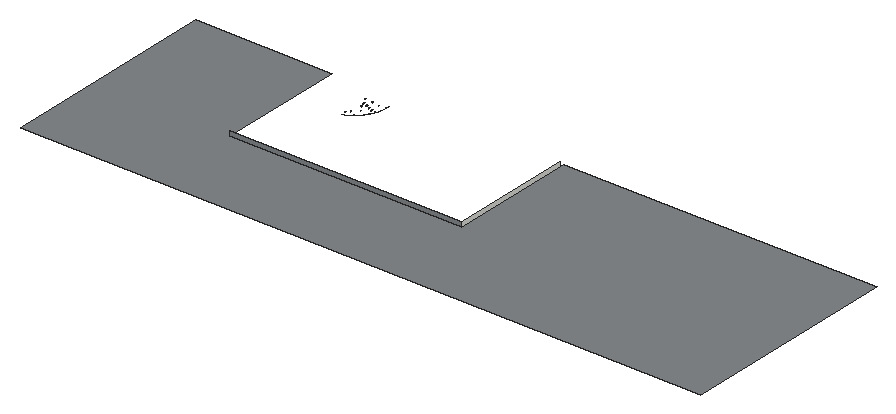
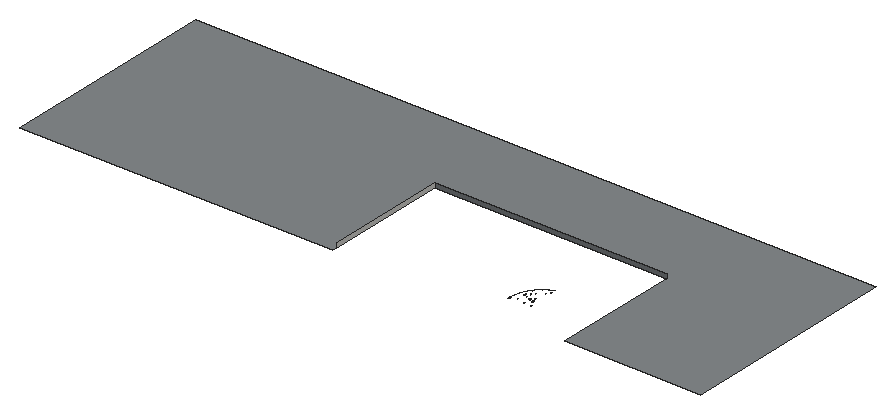
# SketchUp Ruby script. Lengths in inches.
U = 1.inch
M = Sketchup.active_model
def pt(a) = Geom::Point3d.new(a.map { |v| v * U })
def face(e, loops, mat)
  f = e.add_face(loops[0].map { |a| pt(a) })
  loops[1..].each { |l| e.add_face(l.map { |a| pt(a) }).erase! }
  f.material = f.back_material = mat if mat
  f
end
# faces: each face lists its corners as indices into pts; further lists are holes
def faces(e, pts, list, mat = nil) = list.each { |f| face(e, (f[0].is_a?(Array) ? f : [f]).map { |l| l.map { |i| pts[i] } }, mat) }
# xy, xz, yz: faces in a plane at the given z, y or x. An outline is a flat list of corners, or four numbers for a rectangle; further outlines are holes
def ring(l) = l.size == 4 ? [[l[0], l[1]], [l[2], l[1]], [l[2], l[3]], [l[0], l[3]]] : l.each_slice(2).to_a
def flat(e, list, mat, &to3) = list.each { |f| face(e, (f[0].is_a?(Array) ? f : [f]).map { |l| ring(l).map { |u, v| to3.(u, v) } }, mat) }
def xy(e, z, list, mat = nil) = flat(e, list, mat) { |x, y| [x, y, z] }
def xz(e, y, list, mat = nil) = flat(e, list, mat) { |x, z| [x, y, z] }
def yz(e, x, list, mat = nil) = flat(e, list, mat) { |y, z| [x, y, z] }
def lines(e, pts, list) = list.each { |a, b| e.add_line(pt(pts[a]), pt(pts[b])) }
# prism: a flat outline (further loops are holes) pulled along v
def prism(e, loops, v, mat = nil)
  f = face(e, loops, mat); d = Geom::Vector3d.new(v.map { |x| x * U })
  f.pushpull(f.normal.samedirection?(d) ? d.length : -d.length)
end
def box(e, o, s, mat = nil) = prism(e, [[o, [o[0] + s[0], o[1], o[2]], [o[0] + s[0], o[1] + s[1], o[2]], [o[0], o[1] + s[1], o[2]]]], [0, 0, s[2]], mat)
def at(x, y, z, deg = 0) = Geom::Transformation.translation(pt([x, y, z])) * Geom::Transformation.rotation(ORIGIN, Z_AXIS, deg.degrees)
def axes(o, x, y, z) = Geom::Transformation.new([*x, 0, *y, 0, *z, 0, *pt(o).to_a, 1])
def part(name) = M.definitions.add(name)
# library, detail: a bought-in or finely detailed component or shape, given as its bounding box
def library(name, o, s) = part(name).tap { |d| box(d.entities, o, s) }
def detail(e, o, s) = box(e.add_group.entities, o, s)
def put(e, d, t, mat = nil) = e.add_instance(d, t).tap { |i| i.material = mat if mat }
def group(e, t, mat = nil) = e.add_group.tap { |g| g.transformation = t; g.material = mat if mat }.entities
root = M.entities
M.materials.add("[Asphalt_Stamped_Brick]").color = [149, 133, 134]
M.materials.add("[Blacktop Old 01]").color = [132, 136, 139]
M.materials.add("[Metal_Steel_Textured_White]").color = [191, 191, 191]
xy(root,0,[[4.25,0,4.25,181.5,116.615,181.5,116.615,76.29,308.325,76.29,308.325,181.5,566.5625,181.5,566.5625,0]],"[Blacktop Old 01]")
xy(root,3.625,[[165.877,142.641,165.872,142.643,165.868,142.647,165.865,142.651,165.863,142.656,165.862,142.661,165.863,142.666,165.865,142.671,165.868,142.675,165.872,142.678,165.877,142.68,165.882,142.681,165.887,142.68,165.892,142.678,165.896,142.675,165.899,142.671,165.901,142.666,165.902,142.661,165.901,142.656,165.899,142.651,165.896,142.647,165.892,142.643,165.887,142.641],[170.535,147.293,170.529,147.294,170.525,147.296,170.521,147.299,170.517,147.303,170.515,147.308,170.515,147.318,170.517,147.323,170.521,147.327,170.525,147.33,170.529,147.332,170.535,147.333,170.54,147.332,170.545,147.33,170.549,147.327,170.552,147.323,170.554,147.318,170.555,147.313,170.554,147.308,170.552,147.303,170.549,147.299,170.545,147.296,170.54,147.294],[162.784,154.587,162.779,154.588,162.774,154.59,162.77,154.593,162.767,154.597,162.765,154.602,162.764,154.607,162.765,154.613,162.767,154.617,162.77,154.621,162.774,154.625,162.779,154.627,162.789,154.627,162.794,154.625,162.798,154.621,162.801,154.617,162.803,154.613,162.804,154.607,162.803,154.602,162.801,154.597,162.798,154.593,162.794,154.59,162.789,154.588],[162.103,155.035,162.097,155.036,162.093,155.038,162.089,155.041,162.085,155.045,162.083,155.05,162.083,155.06,162.085,155.065,162.089,155.069,162.093,155.072,162.097,155.074,162.103,155.075,162.108,155.074,162.113,155.072,162.117,155.069,162.12,155.065,162.122,155.06,162.123,155.055,162.122,155.05,162.12,155.045,162.117,155.041,162.113,155.038,162.108,155.036],[168.183,156.181,168.178,156.183,168.174,156.186,168.17,156.191,168.168,156.195,168.168,156.206,168.17,156.21,168.174,156.215,168.178,156.218,168.183,156.22,168.193,156.22,168.198,156.218,168.202,156.215,168.205,156.21,168.207,156.206,168.208,156.2,168.207,156.195,168.205,156.191,168.202,156.186,168.198,156.183,168.193,156.181],
  [165.188,157.423,165.183,157.424,165.178,157.426,165.174,157.429,165.171,157.433,165.169,157.438,165.168,157.443,165.169,157.448,165.171,157.453,165.174,157.457,165.178,157.46,165.183,157.462,165.188,157.463,165.193,157.462,165.198,157.46,165.202,157.457,165.205,157.453,165.207,157.448,165.208,157.443,165.207,157.438,165.205,157.433,165.202,157.429,165.198,157.426,165.193,157.424],[161.18,158.219,161.175,158.22,161.17,158.222,161.166,158.225,161.163,158.229,161.161,158.234,161.16,158.239,161.161,158.244,161.163,158.249,161.166,158.253,161.17,158.256,161.175,158.258,161.18,158.259,161.185,158.258,161.19,158.256,161.194,158.253,161.197,158.249,161.199,158.244,161.2,158.239,161.199,158.234,161.197,158.229,161.194,158.225,161.19,158.222,161.185,158.22],[161.48,158.957,161.476,158.959,161.471,158.963,161.468,158.967,161.466,158.971,161.466,158.982,161.468,158.987,161.471,158.991,161.476,158.994,161.48,158.996,161.486,158.997,161.491,158.996,161.496,158.994,161.5,158.991,161.503,158.987,161.505,158.982,161.506,158.977,161.505,158.971,161.503,158.967,161.5,158.963,161.496,158.959,161.491,158.957]],"[Asphalt_Stamped_Brick]")
xy(root,3.625,[[[159.48,138.919,159.457,138.922,159.436,138.931,159.417,138.945,159.403,138.963,159.394,138.985,159.391,139.008,159.394,139.031,159.403,139.052,159.417,139.071,159.436,139.085,159.457,139.094,159.48,139.097,159.503,139.094,159.525,139.085,159.543,139.071,159.557,139.052,159.566,139.031,159.569,139.008,159.566,138.985,159.557,138.963,159.543,138.945,159.525,138.931,159.503,138.922],[159.48,138.92,159.503,138.923,159.524,138.932,159.542,138.945,159.556,138.964,159.565,138.985,159.568,139.008,159.565,139.03,159.556,139.052,159.542,139.07,159.524,139.084,159.503,139.093,159.48,139.096,159.457,139.093,159.436,139.084,159.418,139.07,159.404,139.052,159.395,139.03,159.392,139.008,159.395,138.985,159.404,138.964,159.418,138.945,159.436,138.932,159.457,138.923]],[[160.218,139.224,160.195,139.227,160.173,139.236,160.155,139.25,160.141,139.269,160.132,139.29,160.129,139.313,160.132,139.336,160.141,139.358,160.155,139.376,160.173,139.39,160.195,139.399,160.218,139.402,160.241,139.399,160.262,139.39,160.281,139.376,160.295,139.358,160.304,139.336,160.307,139.313,160.304,139.29,160.295,139.269,160.281,139.25,160.262,139.236,160.241,139.227],[160.218,139.225,160.24,139.228,160.262,139.237,160.28,139.251,160.294,139.269,160.303,139.29,160.306,139.313,160.303,139.336,160.294,139.357,160.28,139.375,160.262,139.389,160.24,139.398,160.218,139.401,160.195,139.398,160.174,139.389,160.156,139.375,160.142,139.357,160.133,139.336,160.13,139.313,160.133,139.29,160.142,139.269,160.156,139.251,160.174,139.237,160.195,139.228]],[[163.155,140.772,163.146,140.773,163.137,140.777,163.13,140.783,163.124,140.79,163.12,140.799,163.119,140.809,163.12,140.818,163.124,140.827,163.13,140.834,163.137,140.84,163.146,140.844,163.155,140.845,163.165,140.844,163.174,140.84,163.181,140.834,163.187,140.827,163.191,140.818,163.192,140.809,163.191,140.799,163.187,140.79,163.181,140.783,163.174,140.777,163.165,140.773],[163.15,140.789,163.161,140.789,163.165,140.791,163.169,140.794,163.173,140.799,163.175,140.803,163.175,140.814,163.173,140.819,163.169,140.823,163.165,140.826,163.161,140.828,163.15,140.828,163.145,140.826,163.141,140.823,163.138,140.819,163.136,140.814,163.135,140.809,163.136,140.803,163.138,140.799,163.141,140.794,163.145,140.791]],[[158.975,142.224,158.952,142.227,158.931,142.236,158.912,142.25,158.898,142.269,158.889,142.29,158.886,142.313,158.889,142.336,158.898,142.358,158.912,142.376,158.931,142.39,158.952,142.399,158.975,142.402,158.998,142.399,159.02,142.39,159.038,142.376,159.052,142.358,159.061,142.336,159.064,142.313,159.061,142.29,159.052,142.269,159.038,142.25,159.02,142.236,158.998,142.227],[158.975,142.225,158.998,142.228,159.019,142.237,159.037,142.251,159.051,142.269,159.06,142.29,159.063,142.313,159.06,142.336,159.051,142.357,159.037,142.375,159.019,142.389,158.998,142.398,158.975,142.401,158.952,142.398,158.931,142.389,158.913,142.375,158.899,142.357,158.89,142.336,158.887,142.313,158.89,142.29,158.899,142.269,158.913,142.251,158.931,142.237,158.952,142.228]],[[165.882,142.624,165.873,142.625,165.864,142.629,165.856,142.635,165.85,142.642,165.847,142.651,165.846,142.661,165.847,142.67,165.85,142.679,165.856,142.687,165.864,142.692,165.873,142.696,165.882,142.697,165.892,142.696,165.9,142.692,165.908,142.687,165.914,142.679,165.917,142.67,165.919,142.661,165.917,142.651,165.914,142.642,165.908,142.635,165.9,142.629,165.892,142.625],[165.877,142.641,165.887,142.641,165.892,142.643,165.896,142.647,165.899,142.651,165.901,142.656,165.902,142.661,165.901,142.666,165.899,142.671,165.896,142.675,165.892,142.678,165.887,142.68,165.882,142.681,165.877,142.68,165.872,142.678,165.868,142.675,165.865,142.671,165.863,142.666,165.862,142.661,165.863,142.656,165.865,142.651,165.868,142.647,165.872,142.643]],
  [[168.355,144.751,168.332,144.755,168.31,144.763,168.292,144.778,168.278,144.796,168.269,144.817,168.266,144.84,168.269,144.863,168.278,144.885,168.292,144.903,168.31,144.917,168.332,144.926,168.355,144.929,168.378,144.926,168.399,144.917,168.418,144.903,168.432,144.885,168.441,144.863,168.444,144.84,168.441,144.817,168.432,144.796,168.418,144.778,168.399,144.763,168.378,144.755],[168.355,144.752,168.378,144.755,168.399,144.764,168.417,144.778,168.431,144.796,168.44,144.818,168.443,144.84,168.44,144.863,168.431,144.884,168.417,144.903,168.399,144.917,168.378,144.925,168.355,144.928,168.332,144.925,168.311,144.917,168.293,144.903,168.279,144.884,168.27,144.863,168.267,144.84,168.27,144.818,168.279,144.796,168.293,144.778,168.311,144.764,168.332,144.755]],[[161.174,144.911,161.151,144.914,161.13,144.922,161.111,144.936,161.097,144.955,161.089,144.976,161.086,144.999,161.089,145.021,161.097,145.043,161.111,145.061,161.13,145.075,161.151,145.083,161.174,145.086,161.196,145.083,161.218,145.075,161.236,145.061,161.25,145.043,161.258,145.021,161.261,144.999,161.258,144.976,161.25,144.955,161.236,144.936,161.218,144.922,161.196,144.914],[161.174,144.962,161.183,144.963,161.192,144.967,161.199,144.973,161.205,144.98,161.209,144.989,161.21,144.999,161.209,145.008,161.205,145.017,161.199,145.024,161.192,145.03,161.183,145.034,161.174,145.035,161.164,145.034,161.155,145.03,161.148,145.024,161.142,145.017,161.138,145.008,161.137,144.999,161.138,144.989,161.142,144.98,161.148,144.973,161.155,144.967,161.164,144.963]],[[161.174,144.962,161.164,144.963,161.155,144.967,161.148,144.973,161.142,144.98,161.138,144.989,161.137,144.999,161.138,145.008,161.142,145.017,161.148,145.024,161.155,145.03,161.164,145.034,161.174,145.035,161.183,145.034,161.192,145.03,161.199,145.024,161.205,145.017,161.209,145.008,161.21,144.999,161.209,144.989,161.205,144.98,161.199,144.973,161.192,144.967,161.183,144.963],[161.168,144.979,161.179,144.979,161.184,144.981,161.1875,144.984,161.191,144.989,161.193,144.993,161.194,144.999,161.193,145.004,161.191,145.009,161.1875,145.013,161.184,145.016,161.179,145.018,161.174,145.019,161.168,145.018,161.164,145.016,161.159,145.013,161.156,145.009,161.154,145.004,161.154,144.993,161.156,144.989,161.159,144.984,161.164,144.981]],[161.168,144.979,161.164,144.981,161.159,144.984,161.156,144.989,161.154,144.993,161.154,145.004,161.156,145.009,161.159,145.013,161.164,145.016,161.168,145.018,161.174,145.019,161.179,145.018,161.184,145.016,161.1875,145.013,161.191,145.009,161.193,145.004,161.194,144.999,161.193,144.993,161.191,144.989,161.1875,144.984,161.184,144.981,161.179,144.979],[[170.535,147.225,170.512,147.228,170.491,147.237,170.472,147.251,170.458,147.269,170.45,147.29,170.447,147.313,170.45,147.336,170.458,147.357,170.472,147.375,170.491,147.389,170.512,147.398,170.535,147.401,170.557,147.398,170.579,147.389,170.597,147.375,170.611,147.357,170.62,147.336,170.623,147.313,170.62,147.29,170.611,147.269,170.597,147.251,170.579,147.237,170.557,147.228],[170.535,147.277,170.544,147.278,170.553,147.281,170.561,147.287,170.566,147.295,170.57,147.304,170.571,147.313,170.57,147.323,170.566,147.331,170.561,147.339,170.553,147.345,170.544,147.349,170.535,147.35,170.525,147.349,170.516,147.345,170.509,147.339,170.503,147.331,170.499,147.323,170.498,147.313,170.499,147.304,170.503,147.295,170.509,147.287,170.516,147.281,170.525,147.278]],
  [[170.535,147.277,170.525,147.278,170.516,147.281,170.509,147.287,170.503,147.295,170.499,147.304,170.498,147.313,170.499,147.323,170.503,147.331,170.509,147.339,170.516,147.345,170.525,147.349,170.535,147.35,170.544,147.349,170.553,147.345,170.561,147.339,170.566,147.331,170.57,147.323,170.571,147.313,170.57,147.304,170.566,147.295,170.561,147.287,170.553,147.281,170.544,147.278],[170.535,147.293,170.54,147.294,170.545,147.296,170.549,147.299,170.552,147.303,170.554,147.308,170.555,147.313,170.554,147.318,170.552,147.323,170.549,147.327,170.545,147.33,170.54,147.332,170.535,147.333,170.529,147.332,170.525,147.33,170.521,147.327,170.517,147.323,170.515,147.318,170.515,147.308,170.517,147.303,170.521,147.299,170.525,147.296,170.529,147.294]],[[165.856,149.593,165.833,149.596,165.812,149.605,165.794,149.619,165.78,149.637,165.771,149.658,165.768,149.681,165.771,149.703,165.78,149.725,165.794,149.743,165.812,149.757,165.833,149.766,165.856,149.769,165.878,149.766,165.9,149.757,165.918,149.743,165.932,149.725,165.941,149.703,165.944,149.681,165.941,149.658,165.932,149.637,165.918,149.619,165.9,149.605,165.878,149.596],[165.856,149.644,165.865,149.645,165.874,149.649,165.882,149.655,165.887,149.662,165.891,149.671,165.892,149.681,165.891,149.69,165.887,149.699,165.882,149.707,165.874,149.712,165.865,149.716,165.856,149.717,165.846,149.716,165.837,149.712,165.83,149.707,165.824,149.699,165.82,149.69,165.819,149.681,165.82,149.671,165.824,149.662,165.83,149.655,165.837,149.649,165.846,149.645]],[[165.856,149.644,165.846,149.645,165.837,149.649,165.83,149.655,165.824,149.662,165.82,149.671,165.819,149.681,165.82,149.69,165.824,149.699,165.83,149.707,165.837,149.712,165.846,149.716,165.856,149.717,165.865,149.716,165.874,149.712,165.882,149.707,165.887,149.699,165.891,149.69,165.892,149.681,165.891,149.671,165.887,149.662,165.882,149.655,165.874,149.649,165.865,149.645],[165.851,149.661,165.861,149.661,165.866,149.663,165.87,149.667,165.873,149.671,165.875,149.676,165.876,149.681,165.875,149.686,165.873,149.691,165.87,149.695,165.866,149.698,165.861,149.7,165.856,149.701,165.851,149.7,165.846,149.698,165.842,149.695,165.838,149.691,165.836,149.686,165.836,149.676,165.838,149.671,165.846,149.663]],[165.851,149.661,165.846,149.663,165.838,149.671,165.836,149.676,165.836,149.686,165.838,149.691,165.842,149.695,165.846,149.698,165.851,149.7,165.856,149.701,165.861,149.7,165.866,149.698,165.87,149.695,165.873,149.691,165.875,149.686,165.876,149.681,165.875,149.676,165.873,149.671,165.87,149.667,165.866,149.663,165.861,149.661],[[172.387,149.951,172.364,149.954,172.342,149.963,172.324,149.977,172.31,149.995,172.301,150.017,172.298,150.04,172.301,150.063,172.31,150.084,172.324,150.103,172.342,150.117,172.364,150.126,172.387,150.129,172.41,150.126,172.431,150.117,172.45,150.103,172.464,150.084,172.473,150.063,172.476,150.04,172.473,150.017,172.464,149.995,172.45,149.977,172.431,149.963,172.41,149.954],[172.387,149.952,172.41,149.955,172.431,149.964,172.449,149.978,172.463,149.996,172.472,150.017,172.475,150.04,172.472,150.0625,172.463,150.084,172.449,150.102,172.431,150.116,172.41,150.125,172.387,150.128,172.364,150.125,172.343,150.116,172.325,150.102,172.311,150.084,172.302,150.0625,172.299,150.04,172.302,150.017,172.311,149.996,172.325,149.978,172.343,149.964,172.364,149.955]],
  [[172.387,150.003,172.377,150.005,172.368,150.008,172.361,150.014,172.355,150.022,172.351,150.03,172.35,150.04,172.351,150.049,172.355,150.058,172.361,150.066,172.368,150.072,172.377,150.075,172.387,150.077,172.396,150.075,172.405,150.072,172.413,150.066,172.418,150.058,172.422,150.049,172.423,150.04,172.422,150.03,172.418,150.022,172.413,150.014,172.405,150.008,172.396,150.005],[172.387,150.02,172.392,150.021,172.397,150.023,172.401,150.026,172.404,150.03,172.406,150.035,172.407,150.04,172.406,150.045,172.404,150.05,172.401,150.054,172.397,150.057,172.392,150.059,172.387,150.06,172.382,150.059,172.377,150.057,172.373,150.054,172.37,150.05,172.368,150.045,172.367,150.04,172.368,150.035,172.37,150.03,172.373,150.026,172.377,150.023,172.382,150.021]],[172.387,150.02,172.382,150.021,172.377,150.023,172.373,150.026,172.37,150.03,172.368,150.035,172.367,150.04,172.368,150.045,172.37,150.05,172.373,150.054,172.377,150.057,172.382,150.059,172.387,150.06,172.392,150.059,172.397,150.057,172.401,150.054,172.404,150.05,172.406,150.045,172.407,150.04,172.406,150.035,172.404,150.03,172.401,150.026,172.397,150.023,172.392,150.021],[[168.197,151.933,168.174,151.936,168.152,151.945,168.134,151.959,168.12,151.977,168.111,151.999,168.108,152.022,168.111,152.045,168.12,152.066,168.134,152.085,168.152,152.099,168.174,152.108,168.197,152.111,168.22,152.108,168.241,152.099,168.26,152.085,168.274,152.066,168.283,152.045,168.286,152.022,168.283,151.999,168.274,151.977,168.26,151.959,168.241,151.945,168.22,151.936],[168.197,151.934,168.22,151.937,168.241,151.946,168.259,151.96,168.273,151.978,168.282,151.999,168.285,152.022,168.282,152.045,168.273,152.066,168.259,152.084,168.241,152.098,168.22,152.107,168.197,152.11,168.174,152.107,168.153,152.098,168.135,152.084,168.121,152.066,168.112,152.045,168.109,152.022,168.112,151.999,168.121,151.978,168.135,151.96,168.153,151.946,168.174,151.937]],[[168.197,151.985,168.187,151.986,168.178,151.99,168.171,151.996,168.165,152.003,168.161,152.012,168.16,152.022,168.161,152.031,168.165,152.04,168.171,152.048,168.178,152.053,168.187,152.057,168.197,152.058,168.206,152.057,168.215,152.053,168.223,152.048,168.228,152.04,168.232,152.031,168.233,152.022,168.232,152.012,168.228,152.003,168.223,151.996,168.215,151.99,168.206,151.986],[168.192,152.002,168.202,152.002,168.207,152.004,168.211,152.008,168.214,152.012,168.216,152.017,168.217,152.022,168.216,152.027,168.214,152.032,168.211,152.036,168.207,152.039,168.202,152.041,168.197,152.042,168.192,152.041,168.187,152.039,168.183,152.036,168.179,152.032,168.177,152.027,168.177,152.017,168.179,152.012,168.187,152.004]],[[173.882,152.89,173.859,152.893,173.838,152.901,173.82,152.915,173.806,152.934,173.797,152.955,173.794,152.978,173.797,153,173.806,153.022,173.82,153.04,173.838,153.054,173.859,153.0625,173.882,153.066,173.905,153.0625,173.926,153.054,173.944,153.04,173.958,153.022,173.967,153,173.97,152.978,173.967,152.955,173.958,152.934,173.944,152.915,173.926,152.901,173.905,152.893],[173.882,152.941,173.892,152.942,173.9,152.946,173.908,152.952,173.914,152.959,173.917,152.968,173.919,152.978,173.917,152.987,173.914,152.996,173.908,153.003,173.9,153.009,173.892,153.013,173.882,153.014,173.873,153.013,173.864,153.009,173.856,153.003,173.85,152.996,173.847,152.987,173.846,152.978,173.847,152.968,173.85,152.959,173.856,152.952,173.864,152.946,173.873,152.942]],
  [[174.1875,153.626,174.165,153.629,174.143,153.638,174.125,153.652,174.111,153.671,174.102,153.692,174.099,153.715,174.102,153.738,174.111,153.76,174.125,153.778,174.143,153.792,174.165,153.801,174.1875,153.804,174.211,153.801,174.232,153.792,174.251,153.778,174.265,153.76,174.274,153.738,174.277,153.715,174.274,153.692,174.265,153.671,174.251,153.652,174.232,153.638,174.211,153.629],[174.1875,153.627,174.21,153.63,174.232,153.639,174.25,153.653,174.264,153.671,174.273,153.692,174.276,153.715,174.273,153.738,174.264,153.759,174.25,153.777,174.232,153.791,174.21,153.8,174.1875,153.803,174.165,153.8,174.144,153.791,174.125,153.777,174.112,153.759,174.103,153.738,174.1,153.715,174.103,153.692,174.112,153.671,174.125,153.653,174.144,153.639,174.165,153.63]],[[174.1875,153.627,174.165,153.63,174.144,153.639,174.125,153.653,174.112,153.671,174.103,153.692,174.1,153.715,174.103,153.738,174.112,153.759,174.125,153.777,174.144,153.791,174.165,153.8,174.1875,153.803,174.21,153.8,174.232,153.791,174.25,153.777,174.264,153.759,174.273,153.738,174.276,153.715,174.273,153.692,174.264,153.671,174.25,153.653,174.232,153.639,174.21,153.63],[174.1875,153.679,174.197,153.68,174.206,153.684,174.214,153.689,174.219,153.697,174.223,153.706,174.224,153.715,174.223,153.725,174.219,153.734,174.214,153.741,174.206,153.747,174.197,153.751,174.1875,153.752,174.178,153.751,174.169,153.747,174.162,153.741,174.156,153.734,174.152,153.725,174.151,153.715,174.152,153.706,174.156,153.697,174.162,153.689,174.169,153.684,174.178,153.68]],[[174.1875,153.679,174.178,153.68,174.169,153.684,174.162,153.689,174.156,153.697,174.152,153.706,174.151,153.715,174.152,153.725,174.156,153.734,174.162,153.741,174.169,153.747,174.178,153.751,174.1875,153.752,174.197,153.751,174.206,153.747,174.214,153.741,174.219,153.734,174.223,153.725,174.224,153.715,174.223,153.706,174.219,153.697,174.214,153.689,174.206,153.684,174.197,153.68],[174.1875,153.695,174.193,153.696,174.198,153.698,174.202,153.701,174.205,153.705,174.207,153.71,174.208,153.715,174.207,153.72,174.205,153.725,174.202,153.729,174.198,153.733,174.193,153.735,174.183,153.735,174.178,153.733,174.17,153.725,174.168,153.72,174.168,153.71,174.17,153.705,174.174,153.701,174.178,153.698,174.183,153.696]],[[170.882,154.131,170.859,154.134,170.838,154.143,170.819,154.157,170.805,154.176,170.796,154.197,170.793,154.22,170.796,154.243,170.805,154.265,170.819,154.283,170.838,154.297,170.859,154.306,170.882,154.309,170.905,154.306,170.927,154.297,170.945,154.283,170.959,154.265,170.968,154.243,170.971,154.22,170.968,154.197,170.959,154.176,170.945,154.157,170.927,154.143,170.905,154.134],[170.882,154.132,170.905,154.135,170.926,154.144,170.944,154.158,170.958,154.176,170.967,154.197,170.97,154.22,170.967,154.243,170.958,154.264,170.944,154.282,170.926,154.296,170.905,154.305,170.882,154.308,170.859,154.305,170.838,154.296,170.82,154.282,170.806,154.264,170.797,154.243,170.794,154.22,170.797,154.197,170.806,154.176,170.82,154.158,170.838,154.144,170.859,154.135]],[[162.784,154.571,162.775,154.572,162.766,154.576,162.758,154.581,162.752,154.589,162.749,154.598,162.748,154.607,162.749,154.617,162.752,154.626,162.758,154.633,162.766,154.639,162.775,154.643,162.784,154.644,162.794,154.643,162.802,154.639,162.81,154.633,162.816,154.626,162.819,154.617,162.821,154.607,162.819,154.598,162.816,154.589,162.81,154.581,162.802,154.576,162.794,154.572],[162.784,154.587,162.789,154.588,162.794,154.59,162.798,154.593,162.801,154.597,162.803,154.602,162.804,154.607,162.803,154.613,162.801,154.617,162.798,154.621,162.794,154.625,162.789,154.627,162.779,154.627,162.774,154.625,162.77,154.621,162.767,154.617,162.765,154.613,162.764,154.607,162.765,154.602,162.767,154.597,162.77,154.593,162.774,154.59,162.779,154.588]],
  [[171.188,154.869,171.165,154.872,171.143,154.881,171.125,154.895,171.111,154.913,171.102,154.935,171.099,154.958,171.102,154.981,171.111,155.002,171.125,155.021,171.143,155.035,171.165,155.044,171.188,155.047,171.211,155.044,171.232,155.035,171.251,155.021,171.265,155.002,171.274,154.981,171.277,154.958,171.274,154.935,171.265,154.913,171.251,154.895,171.232,154.881,171.211,154.872],[171.188,154.87,171.21,154.873,171.232,154.882,171.25,154.896,171.264,154.914,171.273,154.935,171.276,154.958,171.273,154.981,171.264,155.002,171.25,155.02,171.232,155.034,171.21,155.043,171.188,155.046,171.165,155.043,171.144,155.034,171.126,155.02,171.112,155.002,171.103,154.981,171.1,154.958,171.103,154.935,171.112,154.914,171.126,154.896,171.144,154.882,171.165,154.873]],[[162.103,154.966,162.08,154.969,162.058,154.978,162.04,154.992,162.026,155.011,162.017,155.032,162.014,155.055,162.017,155.078,162.026,155.099,162.04,155.118,162.058,155.132,162.08,155.141,162.103,155.144,162.126,155.141,162.147,155.132,162.165,155.118,162.18,155.099,162.189,155.078,162.192,155.055,162.189,155.032,162.18,155.011,162.165,154.992,162.147,154.978,162.126,154.969],[162.103,154.967,162.125,154.97,162.147,154.979,162.165,154.993,162.179,155.011,162.1875,155.032,162.191,155.055,162.1875,155.078,162.179,155.099,162.165,155.117,162.147,155.131,162.125,155.14,162.103,155.143,162.08,155.14,162.059,155.131,162.04,155.117,162.026,155.099,162.018,155.078,162.015,155.055,162.018,155.032,162.026,155.011,162.04,154.993,162.059,154.979,162.08,154.97]],[[162.103,154.967,162.08,154.97,162.059,154.979,162.04,154.993,162.026,155.011,162.018,155.032,162.015,155.055,162.018,155.078,162.026,155.099,162.04,155.117,162.059,155.131,162.08,155.14,162.103,155.143,162.125,155.14,162.147,155.131,162.165,155.117,162.179,155.099,162.1875,155.078,162.191,155.055,162.1875,155.032,162.179,155.011,162.165,154.993,162.147,154.979,162.125,154.97],[162.103,155.018,162.112,155.02,162.121,155.023,162.129,155.029,162.134,155.037,162.138,155.046,162.139,155.055,162.138,155.064,162.134,155.073,162.129,155.081,162.121,155.087,162.112,155.09,162.103,155.092,162.093,155.09,162.084,155.087,162.077,155.081,162.071,155.073,162.067,155.064,162.066,155.055,162.067,155.046,162.071,155.037,162.077,155.029,162.084,155.023,162.093,155.02]],[[162.103,155.018,162.093,155.02,162.084,155.023,162.077,155.029,162.071,155.037,162.067,155.046,162.066,155.055,162.067,155.064,162.071,155.073,162.077,155.081,162.084,155.087,162.093,155.09,162.103,155.092,162.112,155.09,162.121,155.087,162.129,155.081,162.134,155.073,162.138,155.064,162.139,155.055,162.138,155.046,162.134,155.037,162.129,155.029,162.121,155.023,162.112,155.02],[162.103,155.035,162.108,155.036,162.113,155.038,162.117,155.041,162.12,155.045,162.122,155.05,162.123,155.055,162.122,155.06,162.12,155.065,162.117,155.069,162.113,155.072,162.108,155.074,162.103,155.075,162.097,155.074,162.093,155.072,162.089,155.069,162.085,155.065,162.083,155.06,162.083,155.05,162.085,155.045,162.089,155.041,162.093,155.038,162.097,155.036]],[[167.882,155.374,167.859,155.377,167.838,155.386,167.819,155.4,167.805,155.418,167.796,155.44,167.793,155.463,167.796,155.486,167.805,155.507,167.819,155.526,167.838,155.54,167.859,155.549,167.882,155.552,167.905,155.549,167.927,155.54,167.945,155.526,167.959,155.507,167.968,155.486,167.971,155.463,167.968,155.44,167.959,155.418,167.945,155.4,167.927,155.386,167.905,155.377],[167.882,155.375,167.905,155.378,167.926,155.387,167.944,155.401,167.958,155.419,167.967,155.44,167.97,155.463,167.967,155.486,167.958,155.507,167.944,155.525,167.926,155.539,167.905,155.548,167.882,155.551,167.859,155.548,167.838,155.539,167.82,155.525,167.806,155.507,167.797,155.486,167.794,155.463,167.797,155.44,167.806,155.419,167.82,155.401,167.838,155.387,167.859,155.378]],
  [[168.188,156.112,168.165,156.115,168.143,156.124,168.125,156.138,168.111,156.156,168.102,156.177,168.099,156.2,168.102,156.223,168.111,156.245,168.125,156.263,168.143,156.277,168.165,156.286,168.188,156.289,168.211,156.286,168.232,156.277,168.251,156.263,168.265,156.245,168.274,156.223,168.277,156.2,168.274,156.177,168.265,156.156,168.251,156.138,168.232,156.124,168.211,156.115],[168.188,156.113,168.211,156.116,168.232,156.124,168.25,156.138,168.264,156.157,168.273,156.178,168.276,156.2,168.273,156.223,168.264,156.244,168.25,156.263,168.232,156.277,168.211,156.285,168.188,156.288,168.165,156.285,168.144,156.277,168.126,156.263,168.112,156.244,168.103,156.223,168.1,156.2,168.103,156.178,168.112,156.157,168.126,156.138,168.144,156.124,168.165,156.116]],[[168.188,156.113,168.165,156.116,168.144,156.124,168.126,156.138,168.112,156.157,168.103,156.178,168.1,156.2,168.103,156.223,168.112,156.244,168.126,156.263,168.144,156.277,168.165,156.285,168.188,156.288,168.211,156.285,168.232,156.277,168.25,156.263,168.264,156.244,168.273,156.223,168.276,156.2,168.273,156.178,168.264,156.157,168.25,156.138,168.232,156.124,168.211,156.116],[168.188,156.164,168.197,156.165,168.206,156.169,168.214,156.175,168.219,156.182,168.223,156.191,168.224,156.2,168.223,156.21,168.219,156.219,168.214,156.226,168.206,156.232,168.197,156.236,168.188,156.237,168.178,156.236,168.169,156.232,168.162,156.226,168.156,156.219,168.152,156.21,168.151,156.2,168.152,156.191,168.156,156.182,168.162,156.175,168.169,156.169,168.178,156.165]],[[168.188,156.164,168.178,156.165,168.169,156.169,168.162,156.175,168.156,156.182,168.152,156.191,168.151,156.2,168.152,156.21,168.156,156.219,168.162,156.226,168.169,156.232,168.178,156.236,168.188,156.237,168.197,156.236,168.206,156.232,168.214,156.226,168.219,156.219,168.223,156.21,168.224,156.2,168.223,156.191,168.219,156.182,168.214,156.175,168.206,156.169,168.197,156.165],[168.183,156.181,168.193,156.181,168.198,156.183,168.202,156.186,168.205,156.191,168.207,156.195,168.208,156.2,168.207,156.206,168.205,156.21,168.202,156.215,168.198,156.218,168.193,156.22,168.183,156.22,168.178,156.218,168.174,156.215,168.17,156.21,168.168,156.206,168.168,156.195,168.17,156.191,168.174,156.186,168.178,156.183]],[[164.882,156.617,164.859,156.62,164.838,156.628,164.819,156.643,164.805,156.661,164.796,156.682,164.793,156.705,164.796,156.728,164.805,156.75,164.819,156.768,164.838,156.782,164.859,156.791,164.882,156.794,164.905,156.791,164.927,156.782,164.945,156.768,164.959,156.75,164.968,156.728,164.971,156.705,164.968,156.682,164.959,156.661,164.945,156.643,164.927,156.628,164.905,156.62],[164.882,156.618,164.905,156.621,164.926,156.629,164.944,156.643,164.958,156.661,164.967,156.683,164.97,156.705,164.967,156.728,164.958,156.749,164.944,156.768,164.926,156.782,164.905,156.79,164.882,156.793,164.859,156.79,164.838,156.782,164.82,156.768,164.806,156.749,164.797,156.728,164.794,156.705,164.797,156.683,164.806,156.661,164.82,156.643,164.838,156.629,164.859,156.621]],[[164.882,156.669,164.873,156.67,164.864,156.674,164.856,156.68,164.851,156.687,164.847,156.696,164.846,156.705,164.847,156.715,164.851,156.724,164.856,156.731,164.864,156.737,164.873,156.741,164.882,156.742,164.892,156.741,164.901,156.737,164.908,156.731,164.914,156.724,164.918,156.715,164.919,156.705,164.918,156.696,164.914,156.687,164.908,156.68,164.901,156.674,164.892,156.67],[164.882,156.685,164.887,156.686,164.892,156.688,164.896,156.691,164.9,156.695,164.902,156.7,164.902,156.711,164.9,156.715,164.896,156.72,164.892,156.723,164.887,156.725,164.877,156.725,164.872,156.723,164.868,156.72,164.865,156.715,164.863,156.711,164.862,156.705,164.863,156.7,164.865,156.695,164.868,156.691,164.872,156.688,164.877,156.686]],
  [[164.084,156.947,164.061,156.95,164.039,156.959,164.021,156.973,164.007,156.992,163.998,157.013,163.995,157.036,163.998,157.059,164.007,157.081,164.021,157.099,164.039,157.113,164.061,157.122,164.084,157.125,164.107,157.122,164.128,157.113,164.147,157.099,164.161,157.081,164.17,157.059,164.173,157.036,164.17,157.013,164.161,156.992,164.147,156.973,164.128,156.959,164.107,156.95],[164.084,156.948,164.107,156.951,164.128,156.96,164.146,156.974,164.16,156.992,164.169,157.013,164.172,157.036,164.169,157.059,164.16,157.08,164.146,157.098,164.128,157.112,164.107,157.121,164.084,157.124,164.061,157.121,164.04,157.112,164.022,157.098,164.008,157.08,163.999,157.059,163.996,157.036,163.999,157.013,164.008,156.992,164.022,156.974,164.04,156.96,164.061,156.951]],[[164.084,156.948,164.061,156.951,164.04,156.96,164.022,156.974,164.008,156.992,163.999,157.013,163.996,157.036,163.999,157.059,164.008,157.08,164.022,157.098,164.04,157.112,164.061,157.121,164.084,157.124,164.107,157.121,164.128,157.112,164.146,157.098,164.16,157.08,164.169,157.059,164.172,157.036,164.169,157.013,164.16,156.992,164.146,156.974,164.128,156.96,164.107,156.951],[164.084,157,164.093,157.001,164.102,157.004,164.11,157.01,164.116,157.018,164.119,157.027,164.12,157.036,164.119,157.046,164.116,157.054,164.11,157.062,164.102,157.068,164.093,157.072,164.084,157.073,164.074,157.072,164.066,157.068,164.058,157.062,164.052,157.054,164.048,157.046,164.047,157.036,164.048,157.027,164.052,157.018,164.058,157.01,164.066,157.004,164.074,157.001]],[[164.084,157,164.074,157.001,164.066,157.004,164.058,157.01,164.052,157.018,164.048,157.027,164.047,157.036,164.048,157.046,164.052,157.054,164.058,157.062,164.066,157.068,164.074,157.072,164.084,157.073,164.093,157.072,164.102,157.068,164.11,157.062,164.116,157.054,164.119,157.046,164.12,157.036,164.119,157.027,164.116,157.018,164.11,157.01,164.102,157.004,164.093,157.001],[164.084,157.016,164.089,157.017,164.094,157.019,164.098,157.022,164.101,157.026,164.103,157.031,164.104,157.036,164.103,157.041,164.101,157.046,164.098,157.05,164.094,157.053,164.089,157.055,164.084,157.056,164.079,157.055,164.074,157.053,164.07,157.05,164.067,157.046,164.065,157.041,164.064,157.036,164.065,157.031,164.067,157.026,164.07,157.022,164.074,157.019,164.079,157.017]],[[165.188,157.407,165.178,157.408,165.169,157.411,165.162,157.417,165.156,157.425,165.152,157.434,165.151,157.443,165.152,157.453,165.156,157.461,165.162,157.469,165.169,157.475,165.178,157.478,165.188,157.48,165.197,157.478,165.206,157.475,165.214,157.469,165.219,157.461,165.223,157.453,165.224,157.443,165.223,157.434,165.219,157.425,165.214,157.417,165.206,157.411,165.197,157.408],[165.188,157.423,165.193,157.424,165.198,157.426,165.202,157.429,165.205,157.433,165.207,157.438,165.208,157.443,165.207,157.448,165.205,157.453,165.202,157.457,165.198,157.46,165.193,157.462,165.188,157.463,165.183,157.462,165.178,157.46,165.174,157.457,165.171,157.453,165.169,157.448,165.168,157.443,165.169,157.438,165.171,157.433,165.174,157.429,165.178,157.426,165.183,157.424]],[[164.389,157.685,164.366,157.688,164.345,157.697,164.327,157.711,164.3125,157.729,164.303,157.751,164.3,157.774,164.303,157.797,164.3125,157.818,164.327,157.837,164.345,157.851,164.366,157.86,164.389,157.863,164.412,157.86,164.434,157.851,164.452,157.837,164.466,157.818,164.475,157.797,164.478,157.774,164.475,157.751,164.466,157.729,164.452,157.711,164.434,157.697,164.412,157.688],[164.389,157.686,164.412,157.689,164.433,157.698,164.452,157.712,164.466,157.73,164.474,157.751,164.477,157.774,164.474,157.797,164.466,157.818,164.452,157.836,164.433,157.85,164.412,157.859,164.389,157.862,164.367,157.859,164.345,157.85,164.327,157.836,164.313,157.818,164.304,157.797,164.301,157.774,164.304,157.751,164.313,157.73,164.327,157.712,164.345,157.698,164.367,157.689]],
  [[164.389,157.686,164.367,157.689,164.345,157.698,164.327,157.712,164.313,157.73,164.304,157.751,164.301,157.774,164.304,157.797,164.313,157.818,164.327,157.836,164.345,157.85,164.367,157.859,164.389,157.862,164.412,157.859,164.433,157.85,164.452,157.836,164.466,157.818,164.474,157.797,164.477,157.774,164.474,157.751,164.466,157.73,164.452,157.712,164.433,157.698,164.412,157.689],[164.389,157.737,164.399,157.738,164.408,157.742,164.415,157.748,164.421,157.756,164.425,157.764,164.426,157.774,164.425,157.783,164.421,157.792,164.415,157.8,164.408,157.806,164.399,157.809,164.389,157.81,164.38,157.809,164.371,157.806,164.363,157.8,164.358,157.792,164.354,157.783,164.353,157.774,164.354,157.764,164.358,157.756,164.363,157.748,164.371,157.742,164.38,157.738]],[[164.389,157.737,164.38,157.738,164.371,157.742,164.363,157.748,164.358,157.756,164.354,157.764,164.353,157.774,164.354,157.783,164.358,157.792,164.363,157.8,164.371,157.806,164.38,157.809,164.389,157.81,164.399,157.809,164.408,157.806,164.415,157.8,164.421,157.792,164.425,157.783,164.426,157.774,164.425,157.764,164.421,157.756,164.415,157.748,164.408,157.742,164.399,157.738],[164.389,157.754,164.395,157.755,164.399,157.757,164.403,157.76,164.407,157.764,164.409,157.769,164.409,157.779,164.407,157.784,164.403,157.788,164.399,157.791,164.395,157.793,164.389,157.794,164.384,157.793,164.379,157.791,164.375,157.788,164.372,157.784,164.37,157.779,164.369,157.774,164.37,157.769,164.372,157.764,164.375,157.76,164.379,157.757,164.384,157.755]],[164.389,157.754,164.384,157.755,164.379,157.757,164.375,157.76,164.372,157.764,164.37,157.769,164.369,157.774,164.37,157.779,164.372,157.784,164.375,157.788,164.379,157.791,164.384,157.793,164.389,157.794,164.395,157.793,164.399,157.791,164.403,157.788,164.407,157.784,164.409,157.779,164.409,157.769,164.407,157.764,164.403,157.76,164.399,157.757,164.395,157.755],[[161.18,158.15,161.157,158.153,161.136,158.162,161.117,158.176,161.103,158.195,161.094,158.216,161.091,158.239,161.094,158.262,161.103,158.283,161.117,158.302,161.136,158.316,161.157,158.325,161.18,158.328,161.203,158.325,161.224,158.316,161.243,158.302,161.257,158.283,161.266,158.262,161.269,158.239,161.266,158.216,161.257,158.195,161.243,158.176,161.224,158.162,161.203,158.153],[161.18,158.151,161.203,158.154,161.224,158.163,161.242,158.177,161.256,158.195,161.265,158.216,161.268,158.239,161.265,158.262,161.256,158.283,161.242,158.301,161.224,158.315,161.203,158.324,161.18,158.327,161.157,158.324,161.136,158.315,161.118,158.301,161.104,158.283,161.095,158.262,161.092,158.239,161.095,158.216,161.104,158.195,161.118,158.177,161.136,158.163,161.157,158.154]],[[161.18,158.151,161.157,158.154,161.136,158.163,161.118,158.177,161.104,158.195,161.095,158.216,161.092,158.239,161.095,158.262,161.104,158.283,161.118,158.301,161.136,158.315,161.157,158.324,161.18,158.327,161.203,158.324,161.224,158.315,161.242,158.301,161.256,158.283,161.265,158.262,161.268,158.239,161.265,158.216,161.256,158.195,161.242,158.177,161.224,158.163,161.203,158.154],[161.18,158.202,161.189,158.204,161.198,158.207,161.206,158.213,161.212,158.221,161.215,158.229,161.217,158.239,161.215,158.248,161.212,158.257,161.206,158.265,161.198,158.271,161.189,158.274,161.18,158.276,161.171,158.274,161.162,158.271,161.154,158.265,161.148,158.257,161.145,158.248,161.143,158.239,161.145,158.229,161.148,158.221,161.154,158.213,161.162,158.207,161.171,158.204]],
  [[161.18,158.202,161.171,158.204,161.162,158.207,161.154,158.213,161.148,158.221,161.145,158.229,161.143,158.239,161.145,158.248,161.148,158.257,161.154,158.265,161.162,158.271,161.171,158.274,161.18,158.276,161.189,158.274,161.198,158.271,161.206,158.265,161.212,158.257,161.215,158.248,161.217,158.239,161.215,158.229,161.212,158.221,161.206,158.213,161.198,158.207,161.189,158.204],[161.18,158.219,161.185,158.22,161.19,158.222,161.194,158.225,161.197,158.229,161.199,158.234,161.2,158.239,161.199,158.244,161.197,158.249,161.194,158.253,161.19,158.256,161.185,158.258,161.18,158.259,161.175,158.258,161.17,158.256,161.166,158.253,161.163,158.249,161.161,158.244,161.16,158.239,161.161,158.234,161.163,158.229,161.166,158.225,161.17,158.222,161.175,158.22]],[[170.843,158.375,170.834,158.376,170.825,158.38,170.818,158.385,170.812,158.393,170.808,158.402,170.807,158.411,170.808,158.421,170.812,158.43,170.818,158.437,170.825,158.443,170.834,158.447,170.843,158.448,170.853,158.447,170.862,158.443,170.869,158.437,170.875,158.43,170.879,158.421,170.88,158.411,170.879,158.402,170.875,158.393,170.869,158.385,170.862,158.38,170.853,158.376],[170.843,158.391,170.849,158.392,170.853,158.394,170.858,158.397,170.861,158.401,170.863,158.406,170.863,158.416,170.861,158.421,170.858,158.425,170.853,158.429,170.849,158.431,170.838,158.431,170.833,158.429,170.829,158.425,170.826,158.421,170.824,158.416,170.823,158.411,170.824,158.406,170.826,158.401,170.829,158.397,170.833,158.394,170.838,158.392]],[[161.486,158.888,161.463,158.891,161.441,158.9,161.423,158.914,161.409,158.932,161.4,158.954,161.397,158.977,161.4,159,161.409,159.021,161.423,159.039,161.441,159.054,161.463,159.0625,161.486,159.066,161.509,159.0625,161.53,159.054,161.548,159.039,161.5625,159.021,161.571,159,161.574,158.977,161.571,158.954,161.5625,158.932,161.548,158.914,161.53,158.9,161.509,158.891],[161.486,158.889,161.508,158.892,161.53,158.9,161.548,158.914,161.562,158.933,161.57,158.954,161.573,158.977,161.57,158.999,161.562,159.021,161.548,159.039,161.53,159.053,161.508,159.062,161.486,159.065,161.463,159.062,161.442,159.053,161.423,159.039,161.409,159.021,161.401,158.999,161.398,158.977,161.401,158.954,161.409,158.933,161.423,158.914,161.442,158.9,161.463,158.892]],[[161.486,158.889,161.463,158.892,161.442,158.9,161.423,158.914,161.409,158.933,161.401,158.954,161.398,158.977,161.401,158.999,161.409,159.021,161.423,159.039,161.442,159.053,161.463,159.062,161.486,159.065,161.508,159.062,161.53,159.053,161.548,159.039,161.562,159.021,161.57,158.999,161.573,158.977,161.57,158.954,161.562,158.933,161.548,158.914,161.53,158.9,161.508,158.892],[161.486,158.94,161.495,158.941,161.504,158.945,161.511,158.951,161.517,158.958,161.521,158.967,161.522,158.977,161.521,158.986,161.517,158.995,161.511,159.002,161.504,159.008,161.495,159.012,161.486,159.013,161.476,159.012,161.467,159.008,161.46,159.002,161.454,158.995,161.45,158.986,161.449,158.977,161.45,158.967,161.454,158.958,161.46,158.951,161.467,158.945,161.476,158.941]],[[161.486,158.94,161.476,158.941,161.467,158.945,161.46,158.951,161.454,158.958,161.45,158.967,161.449,158.977,161.45,158.986,161.454,158.995,161.46,159.002,161.467,159.008,161.476,159.012,161.486,159.013,161.495,159.012,161.504,159.008,161.511,159.002,161.517,158.995,161.521,158.986,161.522,158.977,161.521,158.967,161.517,158.958,161.511,158.951,161.504,158.945,161.495,158.941],[161.48,158.957,161.491,158.957,161.496,158.959,161.5,158.963,161.503,158.967,161.505,158.971,161.506,158.977,161.505,158.982,161.503,158.987,161.5,158.991,161.496,158.994,161.491,158.996,161.486,158.997,161.48,158.996,161.476,158.994,161.471,158.991,161.468,158.987,161.466,158.982,161.466,158.971,161.468,158.967,161.471,158.963,161.476,158.959]],
  [[158.582,160.091,158.559,160.094,158.538,160.103,158.52,160.117,158.506,160.135,158.497,160.157,158.494,160.179,158.497,160.202,158.506,160.223,158.52,160.242,158.538,160.256,158.559,160.264,158.582,160.267,158.605,160.264,158.626,160.256,158.644,160.242,158.658,160.223,158.667,160.202,158.67,160.179,158.667,160.157,158.658,160.135,158.644,160.117,158.626,160.103,158.605,160.094],[158.582,160.143,158.591,160.144,158.6,160.148,158.608,160.154,158.613,160.161,158.617,160.17,158.618,160.179,158.617,160.189,158.613,160.198,158.608,160.205,158.6,160.211,158.591,160.215,158.582,160.216,158.572,160.215,158.563,160.211,158.556,160.205,158.55,160.198,158.546,160.189,158.545,160.179,158.546,160.17,158.55,160.161,158.556,160.154,158.563,160.148,158.572,160.144]],[[158.582,160.143,158.572,160.144,158.563,160.148,158.556,160.154,158.55,160.161,158.546,160.17,158.545,160.179,158.546,160.189,158.55,160.198,158.556,160.205,158.563,160.211,158.572,160.215,158.582,160.216,158.591,160.215,158.6,160.211,158.608,160.205,158.613,160.198,158.617,160.189,158.618,160.179,158.617,160.17,158.613,160.161,158.608,160.154,158.6,160.148,158.591,160.144],[158.582,160.159,158.587,160.16,158.592,160.162,158.596,160.165,158.599,160.169,158.601,160.174,158.602,160.179,158.601,160.185,158.599,160.189,158.596,160.194,158.592,160.197,158.587,160.199,158.577,160.199,158.572,160.197,158.568,160.194,158.564,160.189,158.5625,160.185,158.562,160.179,158.5625,160.174,158.564,160.169,158.568,160.165,158.572,160.162,158.577,160.16]],[[170.843,161.685,170.834,161.687,170.825,161.69,170.818,161.696,170.812,161.704,170.808,161.713,170.807,161.722,170.808,161.732,170.812,161.74,170.818,161.748,170.825,161.754,170.834,161.757,170.843,161.759,170.853,161.757,170.862,161.754,170.869,161.748,170.875,161.74,170.879,161.732,170.88,161.722,170.879,161.713,170.875,161.704,170.869,161.696,170.862,161.69,170.853,161.687],[170.843,161.702,170.849,161.703,170.853,161.705,170.858,161.708,170.861,161.712,170.863,161.717,170.863,161.727,170.861,161.732,170.858,161.736,170.853,161.739,170.849,161.741,170.843,161.742,170.838,161.741,170.833,161.739,170.829,161.736,170.826,161.732,170.824,161.727,170.823,161.722,170.824,161.717,170.826,161.712,170.829,161.708,170.833,161.705,170.838,161.703]],[170.843,161.702,170.838,161.703,170.833,161.705,170.829,161.708,170.826,161.712,170.824,161.717,170.823,161.722,170.824,161.727,170.826,161.732,170.829,161.736,170.833,161.739,170.838,161.741,170.843,161.742,170.849,161.741,170.853,161.739,170.858,161.736,170.861,161.732,170.863,161.727,170.863,161.717,170.861,161.712,170.858,161.708,170.853,161.705,170.849,161.703],[164.389,163.289,164.367,163.292,164.345,163.301,164.327,163.315,164.313,163.333,164.304,163.355,164.301,163.377,164.353,163.377,164.354,163.368,164.358,163.359,164.363,163.352,164.371,163.346,164.38,163.342,164.389,163.341,164.399,163.342,164.408,163.346,164.415,163.352,164.421,163.359,164.425,163.368,164.426,163.377,164.477,163.377,164.474,163.355,164.466,163.333,164.452,163.315,164.433,163.301,164.412,163.292],
  [165.188,163.289,165.165,163.292,165.144,163.301,165.126,163.315,165.112,163.333,165.103,163.355,165.1,163.377,165.151,163.377,165.152,163.368,165.156,163.359,165.162,163.352,165.169,163.346,165.178,163.342,165.188,163.341,165.197,163.342,165.206,163.346,165.214,163.352,165.219,163.359,165.223,163.368,165.224,163.377,165.276,163.377,165.273,163.355,165.264,163.333,165.25,163.315,165.232,163.301,165.211,163.292],[[176.033,163.289,176.01,163.292,175.989,163.3,175.97,163.315,175.956,163.333,175.947,163.354,175.944,163.377,175.945,163.377,175.948,163.4,175.957,163.421,175.971,163.44,175.989,163.454,176.01,163.462,176.033,163.465,176.056,163.462,176.077,163.454,176.095,163.44,176.109,163.421,176.118,163.4,176.121,163.377,176.122,163.377,176.119,163.354,176.11,163.333,176.096,163.315,176.078,163.3,176.056,163.292],[175.997,163.377,176.013,163.377,176.014,163.383,176.016,163.387,176.019,163.392,176.023,163.395,176.028,163.397,176.038,163.397,176.043,163.395,176.047,163.392,176.051,163.387,176.053,163.383,176.053,163.377,176.07,163.377,176.069,163.387,176.065,163.396,176.059,163.403,176.052,163.409,176.043,163.413,176.033,163.414,176.024,163.413,176.015,163.409,176.007,163.403,176.002,163.396,175.998,163.387],[176.033,163.357,176.038,163.358,176.043,163.36,176.047,163.363,176.051,163.367,176.053,163.372,176.053,163.377,176.013,163.377,176.014,163.372,176.016,163.367,176.019,163.363,176.023,163.36,176.028,163.358]],[176.033,163.289,176.01,163.292,175.989,163.301,175.971,163.315,175.957,163.333,175.948,163.355,175.945,163.377,175.997,163.377,175.998,163.368,176.002,163.359,176.007,163.352,176.015,163.346,176.024,163.342,176.033,163.341,176.043,163.342,176.052,163.346,176.059,163.352,176.065,163.359,176.069,163.368,176.07,163.377,176.121,163.377,176.118,163.355,176.109,163.333,176.095,163.315,176.077,163.301,176.056,163.292],[164.389,163.357,164.384,163.358,164.379,163.36,164.375,163.363,164.372,163.367,164.37,163.372,164.369,163.377,164.409,163.377,164.409,163.372,164.407,163.367,164.403,163.363,164.399,163.36,164.395,163.358],[176.033,163.357,176.028,163.358,176.023,163.36,176.019,163.363,176.016,163.367,176.014,163.372,176.013,163.377,176.053,163.377,176.053,163.372,176.051,163.367,176.047,163.363,176.043,163.36,176.038,163.358],
  [158.697,163.377,158.698,163.387,158.702,163.396,158.708,163.403,158.715,163.409,158.724,163.413,158.734,163.414,158.743,163.413,158.752,163.409,158.76,163.403,158.765,163.396,158.769,163.387,158.77,163.377,158.754,163.377,158.753,163.383,158.751,163.387,158.748,163.392,158.744,163.395,158.739,163.397,158.729,163.397,158.724,163.395,158.72,163.392,158.716,163.387,158.714,163.383,158.714,163.377],[158.714,163.377,158.714,163.383,158.716,163.387,158.72,163.392,158.724,163.395,158.729,163.397,158.739,163.397,158.744,163.395,158.748,163.392,158.751,163.387,158.753,163.383,158.754,163.377],[164.3,163.377,164.303,163.4,164.3125,163.422,164.327,163.44,164.345,163.454,164.366,163.463,164.389,163.466,164.412,163.463,164.434,163.454,164.452,163.44,164.466,163.422,164.475,163.4,164.478,163.377,164.477,163.377,164.474,163.4,164.466,163.421,164.452,163.44,164.433,163.454,164.412,163.462,164.389,163.465,164.367,163.462,164.345,163.454,164.327,163.44,164.313,163.421,164.304,163.4,164.301,163.377],[164.369,163.377,164.37,163.383,164.372,163.387,164.375,163.392,164.379,163.395,164.384,163.397,164.395,163.397,164.399,163.395,164.403,163.392,164.407,163.387,164.409,163.383,164.409,163.377],[165.1,163.377,165.103,163.4,165.112,163.421,165.126,163.44,165.144,163.454,165.165,163.462,165.188,163.465,165.211,163.462,165.232,163.454,165.25,163.44,165.264,163.421,165.273,163.4,165.276,163.377,165.224,163.377,165.223,163.387,165.219,163.396,165.214,163.403,165.206,163.409,165.197,163.413,165.188,163.414,165.178,163.413,165.169,163.409,165.162,163.403,165.156,163.396,165.152,163.387,165.151,163.377],
  [175.997,163.377,175.998,163.387,176.002,163.396,176.007,163.403,176.015,163.409,176.024,163.413,176.033,163.414,176.043,163.413,176.052,163.409,176.059,163.403,176.065,163.396,176.069,163.387,176.07,163.377,176.053,163.377,176.053,163.383,176.051,163.387,176.047,163.392,176.043,163.395,176.038,163.397,176.028,163.397,176.023,163.395,176.019,163.392,176.016,163.387,176.014,163.383,176.013,163.377],[176.013,163.377,176.014,163.383,176.016,163.387,176.019,163.392,176.023,163.395,176.028,163.397,176.038,163.397,176.043,163.395,176.047,163.392,176.051,163.387,176.053,163.383,176.053,163.377],[[170.843,164.945,170.821,164.948,170.799,164.957,170.781,164.971,170.767,164.989,170.758,165.01,170.755,165.033,170.758,165.056,170.767,165.077,170.781,165.095,170.799,165.109,170.821,165.118,170.843,165.121,170.866,165.118,170.887,165.109,170.906,165.095,170.92,165.077,170.928,165.056,170.931,165.033,170.928,165.01,170.92,164.989,170.906,164.971,170.887,164.957,170.866,164.948],[170.843,164.996,170.853,164.997,170.862,165.001,170.869,165.007,170.875,165.015,170.879,165.023,170.88,165.033,170.879,165.042,170.875,165.051,170.869,165.059,170.862,165.065,170.853,165.068,170.843,165.069,170.834,165.068,170.825,165.065,170.818,165.059,170.812,165.051,170.808,165.042,170.807,165.033,170.808,165.023,170.812,165.015,170.818,165.007,170.825,165.001,170.834,164.997]],[[170.843,164.996,170.834,164.997,170.825,165.001,170.818,165.007,170.812,165.015,170.808,165.023,170.807,165.033,170.808,165.042,170.812,165.051,170.818,165.059,170.825,165.065,170.834,165.068,170.843,165.069,170.853,165.068,170.862,165.065,170.869,165.059,170.875,165.051,170.879,165.042,170.88,165.033,170.879,165.023,170.875,165.015,170.869,165.007,170.862,165.001,170.853,164.997],[170.843,165.013,170.849,165.014,170.853,165.016,170.858,165.019,170.861,165.023,170.863,165.028,170.863,165.038,170.861,165.043,170.858,165.047,170.853,165.05,170.849,165.052,170.843,165.053,170.838,165.052,170.833,165.05,170.829,165.047,170.826,165.043,170.824,165.038,170.823,165.033,170.824,165.028,170.826,165.023,170.829,165.019,170.833,165.016,170.838,165.014]]],"[Metal_Steel_Textured_White]")
xz(root,76.29,[[116.615,0,308.325,3.625]],"[Blacktop Old 01]")
yz(root,308.325,[[76.29,0,177.536,3.625]])
p = [[176.566,163.377,3.625],[176.632,163.377,3.625],[176.432,163.377,3.625],[163.125,140.329,3.625],[163.192,140.213,3.625],[163.225,140.156,3.625],
  [165.198,141.413,3.625],[167.054,142.837,3.625],[168.778,144.417,3.625],[170.359,146.142,3.625],[171.783,147.997,3.625],[161.122,139.136,3.625],
  [173.04,149.97,3.625],[176.53,165.714,3.625],[158.989,138.18,3.625],[161.15,139.076,3.625],[174.12,152.045,3.625],[175.015,154.206,3.625],
  [175.718,156.4375,3.625],[176.225,158.721,3.625],[176.53,161.04,3.625],[165.16,141.467,3.625],[167.011,142.888,3.625],[168.731,144.464,3.625],
  [170.308,146.184,3.625],[171.728,148.036,3.625],[172.982,150.004,3.625],[174.059,152.073,3.625],[174.952,154.229,3.625],[175.654,156.455,3.625],
  [176.159,158.733,3.625],[176.464,161.046,3.625],[176.464,165.709,3.625],[158.966,138.243,3.625]]
lines(root,p,[[0,1],[2,0],[3,4],[5,6],[6,7],[7,8],[8,9],[9,10],[11,4],[10,12],[1,13],[14,15],
  [15,5],[12,16],[16,17],[17,18],[18,19],[19,20],[20,1],[5,4],[4,21],[21,22],[22,23],[23,24],
  [24,25],[25,26],[26,27],[27,28],[28,29],[29,30],[30,31],[31,0],[0,32],[33,11]])
